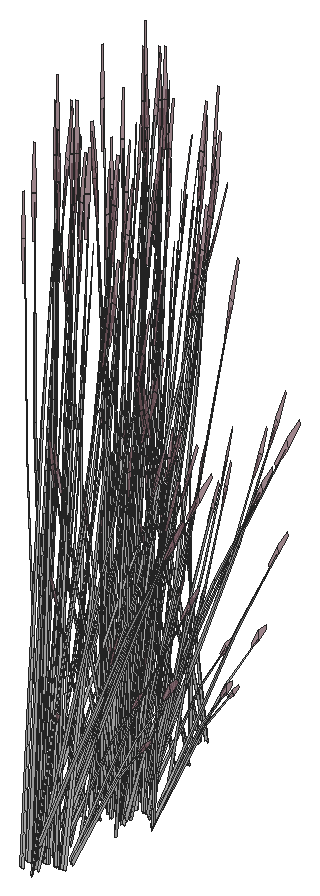
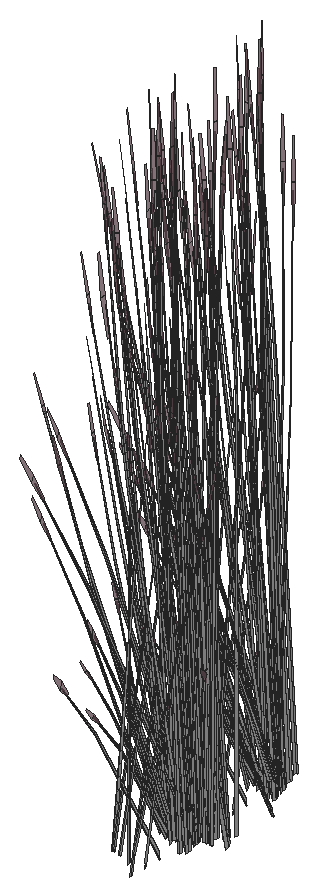
# SketchUp Ruby script. Lengths in inches.
U = 1.inch
M = Sketchup.active_model
def pt(a) = Geom::Point3d.new(a.map { |v| v * U })
def face(e, loops, mat)
  f = e.add_face(loops[0].map { |a| pt(a) })
  loops[1..].each { |l| e.add_face(l.map { |a| pt(a) }).erase! }
  f.material = f.back_material = mat if mat
  f
end
# faces: each face lists its corners as indices into pts; further lists are holes
def faces(e, pts, list, mat = nil) = list.each { |f| face(e, (f[0].is_a?(Array) ? f : [f]).map { |l| l.map { |i| pts[i] } }, mat) }
# xy, xz, yz: faces in a plane at the given z, y or x. An outline is a flat list of corners, or four numbers for a rectangle; further outlines are holes
def ring(l) = l.size == 4 ? [[l[0], l[1]], [l[2], l[1]], [l[2], l[3]], [l[0], l[3]]] : l.each_slice(2).to_a
def flat(e, list, mat, &to3) = list.each { |f| face(e, (f[0].is_a?(Array) ? f : [f]).map { |l| ring(l).map { |u, v| to3.(u, v) } }, mat) }
def xy(e, z, list, mat = nil) = flat(e, list, mat) { |x, y| [x, y, z] }
def xz(e, y, list, mat = nil) = flat(e, list, mat) { |x, z| [x, y, z] }
def yz(e, x, list, mat = nil) = flat(e, list, mat) { |y, z| [x, y, z] }
def lines(e, pts, list) = list.each { |a, b| e.add_line(pt(pts[a]), pt(pts[b])) }
# prism: a flat outline (further loops are holes) pulled along v
def prism(e, loops, v, mat = nil)
  f = face(e, loops, mat); d = Geom::Vector3d.new(v.map { |x| x * U })
  f.pushpull(f.normal.samedirection?(d) ? d.length : -d.length)
end
def box(e, o, s, mat = nil) = prism(e, [[o, [o[0] + s[0], o[1], o[2]], [o[0] + s[0], o[1] + s[1], o[2]], [o[0], o[1] + s[1], o[2]]]], [0, 0, s[2]], mat)
def at(x, y, z, deg = 0) = Geom::Transformation.translation(pt([x, y, z])) * Geom::Transformation.rotation(ORIGIN, Z_AXIS, deg.degrees)
def axes(o, x, y, z) = Geom::Transformation.new([*x, 0, *y, 0, *z, 0, *pt(o).to_a, 1])
def part(name) = M.definitions.add(name)
# library, detail: a bought-in or finely detailed component or shape, given as its bounding box
def library(name, o, s) = part(name).tap { |d| box(d.entities, o, s) }
def detail(e, o, s) = box(e.add_group.entities, o, s)
def put(e, d, t, mat = nil) = e.add_instance(d, t).tap { |i| i.material = mat if mat }
def group(e, t, mat = nil) = e.add_group.tap { |g| g.transformation = t; g.material = mat if mat }.entities
root = M.entities
M.materials.add("LightPink_Translucent").color = [144, 107, 117]
M.materials["LightPink_Translucent"].alpha = 0.75
M.materials.add("[_0053_Ivory_]").color = [200, 200, 200]
c1 = part("blade")
p = [[2.15,0.21,22],[0,0.17,0],[0.09,0.45,0],[2.18,0.31,22],[2.29,0.31,22],[0.38,0.45,0],
  [2.48,0.24,33],[2.49,0.24,33],[2.48,0.22,33]]
faces(c1.entities,p,[[0,1,2,3],[4,5,2,3],[6,3,4,7],[8,0,3,6]])
c2 = part("seeds")
p = [[0.3,-0.1,1.38],[-0.01,-0.03,1.59],[-0.01,-0.03,0.03],[0.14,-0.07,-0.07],[0.29,-0.03,3],[0.15,0.01,3.11]]
faces(c2.entities,p,[[0,1,2,3],[1,0,4,5]],"LightPink_Translucent")
c3 = part("blade with seeds")
put(c3.entities,c1,at(0,0,0))
put(c3.entities,c2,axes([2.4,0.25,30.99],[1.5799,-0.05474,1.17369],[-0.12525,1.92788,0.29478],[-0.07173,-0.02425,1.56792]))
put(root,c3,axes([632.25,312.1,256.18],[0.1831,-0.48359,-0.35414],[0.53419,0.14105,0.4572],[-0.04898,-0.1947,0.87481]),"[_0053_Ivory_]")
put(root,c3,axes([631.36,304.33,254.01],[0.26406,0.70318,0.45755],[-0.7545,0.24452,0.17955],[0.00922,-0.12921,1.58856]),"[_0053_Ivory_]")
put(root,c3,axes([631.24,304.24,253.86],[0.29468,-0.56664,-0.44739],[0.61229,0.27271,0.21531],[0,-0.13062,1.43643]),"[_0053_Ivory_]")
put(root,c3,axes([631.99,295.77,253.86],[-0.19817,-0.54216,0],[0.56587,-0.18986,0],[0,0,1.54371]),"[_0053_Ivory_]")
put(root,c3,axes([631.99,306.0625,253.86],[-0.19817,-0.54216,0],[0.56587,-0.18986,0],[0,0,1.54371]),"[_0053_Ivory_]")
put(root,c3,axes([631.27,296.91,253.15],[0.09829,-0.03422,1.76342],[0.59126,0.18834,-0.26939],[0.01729,0.21228,0.30037]),"[_0053_Ivory_]")
put(root,c3,axes([631.4,297.1,256.18],[-0.1831,0.48359,-0.35414],[-0.53419,-0.14105,0.4572],[0.04898,0.1947,0.87481]),"[_0053_Ivory_]")
put(root,c3,axes([632.79,294.7,253.86],[-0.29468,0.56664,-0.44739],[-0.61229,-0.27271,0.21531],[0,0.13062,1.43643]),"[_0053_Ivory_]")
put(root,c3,axes([632.79,304.99,253.86],[-0.29468,0.56664,-0.44739],[-0.61229,-0.27271,0.21531],[0,0.13062,1.43643]),"[_0053_Ivory_]")
put(root,c3,axes([633.95,294.35,254.13],[-0.47719,-0.45806,0.17642],[0.48088,-0.44429,0.35086],[-0.0527,0.09355,1.60407]),"[_0053_Ivory_]")
put(root,c3,axes([633.95,304.65,254.13],[-0.47719,-0.45806,0.17642],[0.48088,-0.44429,0.35086],[-0.0527,0.09355,1.60407]),"[_0053_Ivory_]")
put(root,c3,axes([632.31,304.38,253.86],[0,-0.72763,0],[0.75945,0,0],[0,0,1.79456]),"[_0053_Ivory_]")
put(root,c3,axes([631.6,304.52,254.09],[0.68433,0.30479,0.24065],[-0.32934,0.63331,0.50002],[0,-0.14599,1.60543]),"[_0053_Ivory_]")
put(root,c3,axes([632.6875,294.38,253.95],[0,0.72727,-0.05637],[-0.75945,0,0],[0,0.02286,1.79368]),"[_0053_Ivory_]")
put(root,c3,axes([632.6875,304.68,253.95],[0,0.72727,-0.05637],[-0.75945,0,0],[0,0.02286,1.79368]),"[_0053_Ivory_]")
put(root,c3,axes([631.38,304.09,254.37],[-0.65953,0.03882,0.44739],[-0.05964,-0.64439,-0.21531],[0.11807,-0.06531,1.43643]),"[_0053_Ivory_]")
put(root,c3,axes([631.07,302.99,254.13],[-0.17545,0.62497,0.17642],[-0.64204,-0.17686,0.35086],[0.11091,-0.00304,1.60407]),"[_0053_Ivory_]")
put(root,c3,axes([632.32,295.79,253.94],[0.26406,0.72244,-0.06012],[-0.7545,0.25315,0],[0.00922,0.02523,1.72173]),"[_0053_Ivory_]")
put(root,c3,axes([632.32,306.08,253.94],[0.26406,0.72244,-0.06012],[-0.7545,0.25315,0],[0.00922,0.02523,1.72173]),"[_0053_Ivory_]")
put(root,c3,axes([630.76,302.22,254.03],[-0.37973,-0.63014,0],[0.6353,-0.35142,-0.51607],[0.14469,-0.08004,1.63711]),"[_0053_Ivory_]")
put(root,c3,axes([631.46,296.67,256.63],[0.28988,0.51132,-0.71045],[-0.59671,0.28496,0.08574],[0.06778,0.24706,1.00501]),"[_0053_Ivory_]")
put(root,c3,axes([634.51,294.84,253.85],[-0.75908,-0.00503,-0.04976],[0,-0.70283,0.49943],[-0.02386,0.16,1.58352]),"[_0053_Ivory_]")
put(root,c3,axes([634.51,305.14,253.85],[-0.75908,-0.00503,-0.04976],[0,-0.70283,0.49943],[-0.02386,0.16,1.58352]),"[_0053_Ivory_]")
put(root,c3,axes([633.01,292.73,254.13],[-0.65264,0.16691,0.17642],[-0.16115,-0.62115,0.35086],[0.05821,0.0905,1.60407]),"[_0053_Ivory_]")
put(root,c3,axes([633.01,303.02,254.13],[-0.65264,0.16691,0.17642],[-0.16115,-0.62115,0.35086],[0.05821,0.0905,1.60407]),"[_0053_Ivory_]")
put(root,c3,axes([632.35,300.69,254.42],[0.07791,0.3667,1.1486],[-0.43222,-0.2031,0.84392],[0.04651,-0.18776,0.25299]),"[_0053_Ivory_]")
put(root,c3,axes([632.35,311.08,254.42],[0.07791,0.3667,1.1486],[-0.43222,-0.2031,0.84392],[0.04651,-0.18776,0.25299]),"[_0053_Ivory_]")
put(root,c3,axes([631.95,303.93,254.01],[-0.50358,0.57069,0.45755],[-0.59827,-0.50377,0.17955],[0.1214,-0.05695,1.58856]),"[_0053_Ivory_]")
put(root,c3,axes([632.81,294.53,253.87],[0.42396,0.40619,0],[-0.42396,0.40619,0],[0,0,1.69266]),"[_0053_Ivory_]")
put(root,c3,axes([632.81,304.83,253.87],[0.42396,0.40619,0],[-0.42396,0.40619,0],[0,0,1.69266]),"[_0053_Ivory_]")
put(root,c3,axes([632.8,294.06,254.37],[0.29468,-0.56664,0.44739],[0.61229,0.27271,-0.21531],[0,0.13062,1.43643]),"[_0053_Ivory_]")
put(root,c3,axes([632.8,304.35,254.37],[0.29468,-0.56664,0.44739],[0.61229,0.27271,-0.21531],[0,0.13062,1.43643]),"[_0053_Ivory_]")
put(root,c3,axes([632.55,296.02,253.86],[0.61229,0.28233,0],[-0.29468,0.58663,0],[0,0,1.74954]),"[_0053_Ivory_]")
put(root,c3,axes([632.55,306.32,253.86],[0.61229,0.28233,0],[-0.29468,0.58663,0],[0,0,1.74954]),"[_0053_Ivory_]")
put(root,c3,axes([631.67,296.77,256.33],[0.59704,0.15764,-0.51099],[-0.20464,0.54049,-0.3958],[0.05475,0.21761,0.97773]),"[_0053_Ivory_]")
put(root,c3,axes([632.6,293.92,254.03],[-0.76764,-0.13249,0.49198],[0.15622,-0.74829,0.19306],[0.11218,0.07226,1.70813]),"[_0053_Ivory_]")
put(root,c3,axes([632.6,304.22,254.03],[-0.76764,-0.13249,0.49198],[0.15622,-0.74829,0.19306],[0.11218,0.07226,1.70813]),"[_0053_Ivory_]")
put(root,c3,axes([634.35,294.94,253.68],[-0.42396,0.39235,-0.30978],[-0.42396,-0.39235,0.30978],[0,0.12637,1.38974]),"[_0053_Ivory_]")
put(root,c3,axes([634.35,305.24,253.68],[-0.42396,0.39235,-0.30978],[-0.42396,-0.39235,0.30978],[0,0.12637,1.38974]),"[_0053_Ivory_]")
put(root,c3,axes([633.14,294.87,253.75],[0.2227,0.57576,-0.69212],[-0.64151,0.20736,-0.18165],[0.02462,0.19497,1.52773]),"[_0053_Ivory_]")
put(root,c3,axes([633.14,305.17,253.75],[0.2227,0.57576,-0.69212],[-0.64151,0.20736,-0.18165],[0.02462,0.19497,1.52773]),"[_0053_Ivory_]")
put(root,c3,axes([632.82,294.25,253.86],[0.67951,0,0],[0,0.65103,0],[0,0,1.78407]),"[_0053_Ivory_]")
put(root,c3,axes([632.82,304.55,253.86],[0.67951,0,0],[0,0.65103,0],[0,0,1.78407]),"[_0053_Ivory_]")
put(root,c3,axes([632.17,303.83,254.37],[-0.36485,-0.52782,0.44739],[0.55265,-0.37168,-0.21531],[0.11807,0.06531,1.43643]),"[_0053_Ivory_]")
put(root,c3,axes([631.5,303.96,254.32],[-0.07077,-0.71755,-0.29095],[0.73712,-0.04339,-0.50002],[0.1298,-0.09558,1.59708]),"[_0053_Ivory_]")
put(root,c3,axes([633.06,294.1875,254.27],[0.56587,-0.18339,0.1448],[0.19817,0.52368,-0.41347],[0,0.11525,1.26744]),"[_0053_Ivory_]")
put(root,c3,axes([633.06,304.48,254.27],[0.56587,-0.18339,0.1448],[0.19817,0.52368,-0.41347],[0,0.11525,1.26744]),"[_0053_Ivory_]")
put(root,c3,axes([633.27,302.46,256.33],[-0.43478,-0.42253,-0.51099],[0.45929,-0.37004,-0.3958],[0.06615,-0.21468,0.97773]),"[_0053_Ivory_]")
put(root,c3,axes([633.27,312.85,256.33],[-0.43478,-0.42253,-0.51099],[0.45929,-0.37004,-0.3958],[0.06615,-0.21468,0.97773]),"[_0053_Ivory_]")
put(root,c3,axes([632.86,294.23,254.32],[0.68399,0.30005,-0.29095],[-0.32934,0.63331,-0.50002],[0.0215,0.15549,1.59708]),"[_0053_Ivory_]")
put(root,c3,axes([632.86,304.52,254.32],[0.68399,0.30005,-0.29095],[-0.32934,0.63331,-0.50002],[0.0215,0.15549,1.59708]),"[_0053_Ivory_]")
put(root,c3,axes([631.41,302.37,253.68],[0.56663,0.1556,-0.30978],[-0.14267,0.54795,0.30978],[0.11423,-0.06319,1.38974]),"[_0053_Ivory_]")
put(root,c3,axes([632.98,301.71,254.24],[-0.17264,0.12729,1.43002],[-0.51703,-0.22279,-0.30754],[0.09584,-0.27707,0.61141]),"[_0053_Ivory_]")
put(root,c3,axes([632.98,312.1,254.24],[-0.17264,0.12729,1.43002],[-0.51703,-0.22279,-0.30754],[0.09584,-0.27707,0.61141]),"[_0053_Ivory_]")
put(root,c3,axes([634.35,294.37,254.13],[0,-0.62885,0.49651],[0.67951,0,0],[0,0.14322,1.57504]),"[_0053_Ivory_]")
put(root,c3,axes([634.35,304.67,254.13],[0,-0.62885,0.49651],[0.67951,0,0],[0,0.14322,1.57504]),"[_0053_Ivory_]")
put(root,c3,axes([634.64,294.96,253.67],[0,0.62885,-0.49651],[-0.67951,0,0],[0,0.14322,1.57504]),"[_0053_Ivory_]")
put(root,c3,axes([634.64,305.25,253.67],[0,0.62885,-0.49651],[-0.67951,0,0],[0,0.14322,1.57504]),"[_0053_Ivory_]")
put(root,c3,axes([631.27,302.12,253.67],[0.56842,-0.31443,-0.49651],[0.33976,0.56381,0],[0.12946,-0.07161,1.57504]),"[_0053_Ivory_]")
put(root,c3,axes([632.01,295.66,255.53],[-0.13883,-0.2019,1.71376],[0.64153,-0.16998,0.13857],[0.14499,0.31697,0.73262]),"[_0053_Ivory_]")
put(root,c3,axes([632.41,303.68,254.27],[0.11717,-0.56122,0.1448],[0.57245,0.09742,-0.41347],[0.10418,0.05763,1.26744]),"[_0053_Ivory_]")
put(root,c3,axes([633.23,302.7,254.13],[-0.56842,-0.31443,0.49651],[0.33976,-0.56381,0],[0.12946,0.07161,1.57504]),"[_0053_Ivory_]")
put(root,c3,axes([633.4,302.65,256.63],[0.0158,-0.58168,-0.71045],[0.66548,0.03907,0.08574],[0.07023,-0.24643,1.00501]),"[_0053_Ivory_]")
put(root,c3,axes([633.4,313.04,256.63],[0.0158,-0.58168,-0.71045],[0.66548,0.03907,0.08574],[0.07023,-0.24643,1.00501]),"[_0053_Ivory_]")
put(root,c3,axes([632.73,295.69,253.84],[0.63764,-0.21337,-0.19198],[0.22406,0.61462,0.00008],[0.07038,-0.02358,1.73897]),"[_0053_Ivory_]")
put(root,c3,axes([632.73,305.99,253.84],[0.63764,-0.21337,-0.19198],[0.22406,0.61462,0.00008],[0.07038,-0.02358,1.73897]),"[_0053_Ivory_]")
put(root,c3,axes([632.74,293.86,253.86],[0.36485,0.52782,-0.44739],[-0.55265,0.37168,0.21531],[0.11807,0.06531,1.43643]),"[_0053_Ivory_]")
put(root,c3,axes([632.74,304.16,253.86],[0.36485,0.52782,-0.44739],[-0.55265,0.37168,0.21531],[0.11807,0.06531,1.43643]),"[_0053_Ivory_]")
put(root,c3,axes([633.68,302.3,256.18],[0.41095,-0.33109,-0.35414],[0.38901,0.37805,0.4572],[0.05919,-0.19208,0.87481]),"[_0053_Ivory_]")
put(root,c3,axes([633.68,312.69,256.18],[0.41095,-0.33109,-0.35414],[0.38901,0.37805,0.4572],[0.05919,-0.19208,0.87481]),"[_0053_Ivory_]")
put(root,c3,axes([633.78,296.26,254.42],[-0.34197,-0.18082,1.1486],[0.44156,-0.18372,0.84392],[0.1191,0.15563,0.25299]),"[_0053_Ivory_]")
put(root,c3,axes([633.78,306.56,254.42],[-0.34197,-0.18082,1.1486],[0.44156,-0.18372,0.84392],[0.1191,0.15563,0.25299]),"[_0053_Ivory_]")
put(root,c3,axes([632.56,296.07,254.24],[0.01072,-0.20846,1.43002],[0.51218,-0.23285,-0.30754],[0.15811,0.2495,0.61141]),"[_0053_Ivory_]")
put(root,c3,axes([631.95,303.41,253.71],[0.40909,-0.47266,-0.62353],[0.50819,0.4286,-0.16365],[0.16393,-0.11791,1.37633]),"[_0053_Ivory_]")
put(root,c3,axes([633.74,292.69,253.68],[0.14267,0.54795,-0.30978],[-0.56663,0.1556,0.30978],[0.11423,0.06319,1.38974]),"[_0053_Ivory_]")
put(root,c3,axes([633.74,302.99,253.68],[0.14267,0.54795,-0.30978],[-0.56663,0.1556,0.30978],[0.11423,0.06319,1.38974]),"[_0053_Ivory_]")
put(root,c3,axes([634.81,294.48,254.03],[0.75945,0,0],[0,0.70283,-0.51607],[0,0.16007,1.63711]),"[_0053_Ivory_]")
put(root,c3,axes([634.81,304.77,254.03],[0.75945,0,0],[0,0.70283,-0.51607],[0,0.16007,1.63711]),"[_0053_Ivory_]")
put(root,c3,axes([632.35,303.86,254.32],[0.61322,-0.4175,-0.29095],[0.40778,0.58992,-0.50002],[0.1513,0.05991,1.59708]),"[_0053_Ivory_]")
put(root,c3,axes([633.83,297.08,254.32],[-0.38947,-0.01972,1.0506],[0.25721,-0.41888,0.58006],[0.15386,0.14882,0.8241]),"[_0053_Ivory_]")
put(root,c3,axes([632.65,302.35,255.53],[-0.11309,0.21615,1.71376],[-0.47441,-0.44731,0.13857],[0.21402,-0.27879,0.73262]),"[_0053_Ivory_]")
put(root,c3,axes([632.65,312.74,255.53],[-0.11309,0.21615,1.71376],[-0.47441,-0.44731,0.13857],[0.21402,-0.27879,0.73262]),"[_0053_Ivory_]")
put(root,c3,axes([630.81,303.49,253.25],[-0.59782,0.25177,1.28929],[-0.19028,-0.72239,0.50096],[0.36709,0.01202,1.46642]),"[_0053_Ivory_]")
put(root,c3,axes([633,296.51,256.33],[0.59932,-0.14948,-0.51099],[0.10484,0.56611,-0.3958],[0.16097,0.16223,0.97773]),"[_0053_Ivory_]")
put(root,c3,axes([633.55,302.375,254.03],[0.37973,-0.63014,0],[0.6353,0.35142,-0.51607],[0.14469,0.08004,1.63711]),"[_0053_Ivory_]")
put(root,c3,axes([634.19,302.1,253.15],[-0.0909,-0.04954,1.76342],[-0.2335,-0.55347,-0.26939],[0.15752,-0.1502,0.30037]),"[_0053_Ivory_]")
put(root,c3,axes([633.9,302.75,253.67],[0.56842,0.31443,-0.49651],[-0.33976,0.56381,0],[0.12946,0.07161,1.57504]),"[_0053_Ivory_]")
put(root,c3,axes([633.87,296.93,253.15],[0.04425,-0.09079,1.76342],[0.55709,-0.26738,-0.26939],[0.16889,0.13839,0.30037]),"[_0053_Ivory_]")
put(root,c3,axes([633.87,307.23,253.15],[0.04425,-0.09079,1.76342],[0.55709,-0.26738,-0.26939],[0.16889,0.13839,0.30037]),"[_0053_Ivory_]")
put(root,c3,axes([634.17,303.43,256.33],[-0.15602,-0.5742,-0.51099],[0.59087,-0.10045,-0.3958],[0.16933,-0.15423,0.97773]),"[_0053_Ivory_]")
put(root,c3,axes([635.21,296.1,255.58],[-0.11624,-0.52862,-0.03492],[0.54943,-0.12153,-0.15832],[0.11473,0.03351,0.52218]),"[_0053_Ivory_]")
put(root,c3,axes([635.21,306.39,255.58],[-0.11624,-0.52862,-0.03492],[0.54943,-0.12153,-0.15832],[0.11473,0.03351,0.52218]),"[_0053_Ivory_]")
put(root,c3,axes([633.07,293.66,253.71],[0.63179,0.1031,-0.62353],[-0.13332,0.63596,-0.16365],[0.18854,0.07706,1.37633]),"[_0053_Ivory_]")
put(root,c3,axes([633.07,303.96,253.71],[0.63179,0.1031,-0.62353],[-0.13332,0.63596,-0.16365],[0.18854,0.07706,1.37633]),"[_0053_Ivory_]")
put(root,c3,axes([635.76,304.33,253.91],[-0.37654,-0.40212,-0.06488],[0.4124,-0.36845,-0.29416],[0.11685,-0.02594,0.97024]),"[_0053_Ivory_]")
put(root,c3,axes([634.9,302.29,254.42],[-0.2023,0.32011,1.1486],[-0.17388,-0.43009,0.84392],[0.16708,-0.10777,0.25299]),"[_0053_Ivory_]")
put(root,c3,axes([632.94,295.03,255.53],[-0.2256,-0.10835,1.71376],[0.46687,-0.45453,0.13857],[0.29098,0.20505,0.73262]),"[_0053_Ivory_]")
put(root,c3,axes([632.94,305.32,255.53],[-0.2256,-0.10835,1.71376],[0.46687,-0.45453,0.13857],[0.29098,0.20505,0.73262]),"[_0053_Ivory_]")
put(root,c3,axes([634.61,303.49,256.18],[0.52868,-0.08987,-0.35414],[0.1396,0.51376,0.4572],[0.1515,-0.13799,0.87481]),"[_0053_Ivory_]")
put(root,c3,axes([634.1875,303.66,256.63],[0.31725,-0.49618,-0.71045],[0.55593,0.35263,0.08574],[0.18942,-0.17977,1.00501]),"[_0053_Ivory_]")
put(root,c3,axes([634.18,296.04,256.18],[0.34557,0.39372,-0.35414],[-0.39459,0.37271,0.4572],[0.20048,0.05671,0.87481]),"[_0053_Ivory_]")
put(root,c3,axes([634.18,306.33,256.18],[0.34557,0.39372,-0.35414],[-0.39459,0.37271,0.4572],[0.20048,0.05671,0.87481]),"[_0053_Ivory_]")
put(root,c3,axes([634.45,304.7,256.33],[0.16454,-0.57202,-0.51099],[0.56413,0.19607,-0.3958],[0.22713,-0.05245,0.97773]),"[_0053_Ivory_]")
put(root,c3,axes([635.86,294.77,254.42],[-0.37526,0.10382,1.1486],[0.17664,-0.42906,0.84392],[0.19907,0.02936,0.25299]),"[_0053_Ivory_]")
put(root,c3,axes([635.86,305.07,254.42],[-0.37526,0.10382,1.1486],[0.17664,-0.42906,0.84392],[0.19907,0.02936,0.25299]),"[_0053_Ivory_]")
put(root,c3,axes([634.65,303.2,254.24],[-0.21697,-0.01863,1.43002],[-0.22228,-0.49966,-0.30754],[0.26655,-0.14135,0.61141]),"[_0053_Ivory_]")
put(root,c3,axes([634.79,304.96,256.18],[0.50475,0.17543,-0.35414],[-0.14722,0.5118,0.4572],[0.20322,-0.04693,0.87481]),"[_0053_Ivory_]")
put(root,c3,axes([633.82,295.77,256.63],[0.60713,0.01514,-0.71045],[-0.04078,0.63759,0.08574],[0.25721,0.06729,1.00501]),"[_0053_Ivory_]")
put(root,c3,axes([633.82,306.07,256.63],[0.60713,0.01514,-0.71045],[-0.04078,0.63759,0.08574],[0.25721,0.06729,1.00501]),"[_0053_Ivory_]")
put(root,c3,axes([635.05,304.86,253.64],[-0.39118,0.07547,1.41583],[-0.06226,-0.6007,0.08104],[0.27398,-0.09092,0.80566]),"[_0053_Ivory_]")
put(root,c3,axes([635.48,304.47,253.15],[-0.03174,-0.09547,1.76342],[0.22015,-0.55846,-0.26939],[0.22208,-0.00803,0.30037]),"[_0053_Ivory_]")
put(root,c3,axes([633.42,294.04,255.53],[-0.25192,0.01424,1.71376],[0.16712,-0.61729,0.13857],[0.35901,0.03818,0.73262]),"[_0053_Ivory_]")
put(root,c3,axes([633.42,304.33,255.53],[-0.25192,0.01424,1.71376],[0.16712,-0.61729,0.13857],[0.35901,0.03818,0.73262]),"[_0053_Ivory_]")
put(root,c3,axes([634.34,304.91,256.63],[0.53369,-0.27773,-0.71045],[0.29743,0.5717,0.08574],[0.25786,-0.06494,1.00501]),"[_0053_Ivory_]")
put(root,c3,axes([635.16,295.46,254.24],[-0.14627,-0.15466,1.43002],[0.19032,-0.51164,-0.30754],[0.29594,0.06931,0.61141]),"[_0053_Ivory_]")
put(root,c3,axes([635.16,305.76,254.24],[-0.14627,-0.15466,1.43002],[0.19032,-0.51164,-0.30754],[0.29594,0.06931,0.61141]),"[_0053_Ivory_]")
